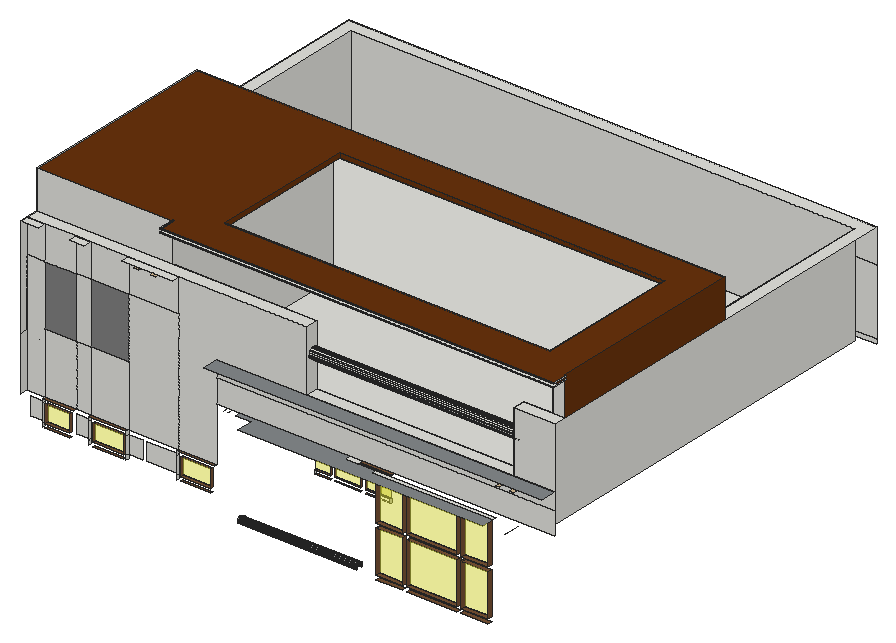
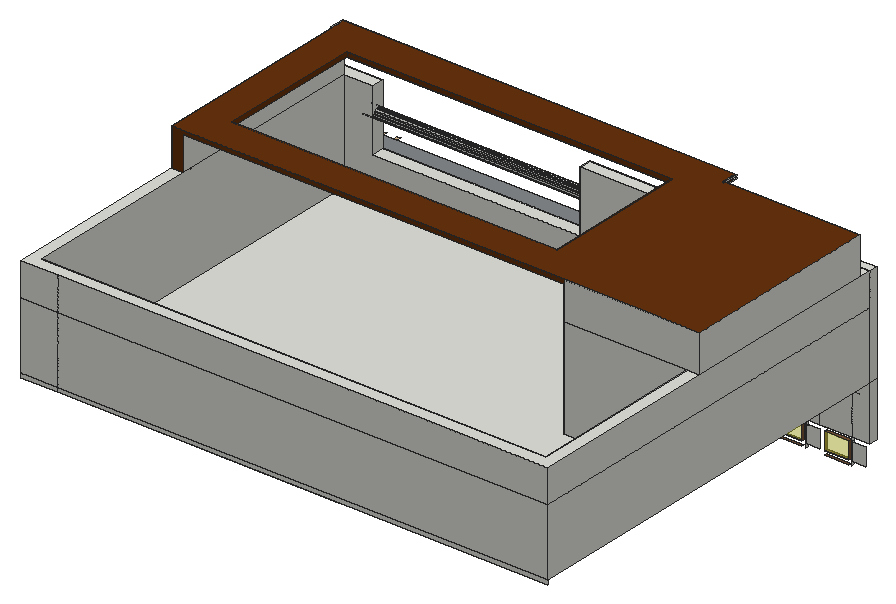
# SketchUp Ruby script. Lengths in inches.
U = 1.inch
M = Sketchup.active_model
def pt(a) = Geom::Point3d.new(a.map { |v| v * U })
def face(e, loops, mat)
  f = e.add_face(loops[0].map { |a| pt(a) })
  loops[1..].each { |l| e.add_face(l.map { |a| pt(a) }).erase! }
  f.material = f.back_material = mat if mat
  f
end
# faces: each face lists its corners as indices into pts; further lists are holes
def faces(e, pts, list, mat = nil) = list.each { |f| face(e, (f[0].is_a?(Array) ? f : [f]).map { |l| l.map { |i| pts[i] } }, mat) }
# xy, xz, yz: faces in a plane at the given z, y or x. An outline is a flat list of corners, or four numbers for a rectangle; further outlines are holes
def ring(l) = l.size == 4 ? [[l[0], l[1]], [l[2], l[1]], [l[2], l[3]], [l[0], l[3]]] : l.each_slice(2).to_a
def flat(e, list, mat, &to3) = list.each { |f| face(e, (f[0].is_a?(Array) ? f : [f]).map { |l| ring(l).map { |u, v| to3.(u, v) } }, mat) }
def xy(e, z, list, mat = nil) = flat(e, list, mat) { |x, y| [x, y, z] }
def xz(e, y, list, mat = nil) = flat(e, list, mat) { |x, z| [x, y, z] }
def yz(e, x, list, mat = nil) = flat(e, list, mat) { |y, z| [x, y, z] }
def lines(e, pts, list) = list.each { |a, b| e.add_line(pt(pts[a]), pt(pts[b])) }
# prism: a flat outline (further loops are holes) pulled along v
def prism(e, loops, v, mat = nil)
  f = face(e, loops, mat); d = Geom::Vector3d.new(v.map { |x| x * U })
  f.pushpull(f.normal.samedirection?(d) ? d.length : -d.length)
end
def box(e, o, s, mat = nil) = prism(e, [[o, [o[0] + s[0], o[1], o[2]], [o[0] + s[0], o[1] + s[1], o[2]], [o[0], o[1] + s[1], o[2]]]], [0, 0, s[2]], mat)
def at(x, y, z, deg = 0) = Geom::Transformation.translation(pt([x, y, z])) * Geom::Transformation.rotation(ORIGIN, Z_AXIS, deg.degrees)
def axes(o, x, y, z) = Geom::Transformation.new([*x, 0, *y, 0, *z, 0, *pt(o).to_a, 1])
def part(name) = M.definitions.add(name)
# library, detail: a bought-in or finely detailed component or shape, given as its bounding box
def library(name, o, s) = part(name).tap { |d| box(d.entities, o, s) }
def detail(e, o, s) = box(e.add_group.entities, o, s)
def put(e, d, t, mat = nil) = e.add_instance(d, t).tap { |i| i.material = mat if mat }
def group(e, t, mat = nil) = e.add_group.tap { |g| g.transformation = t; g.material = mat if mat }.entities
root = M.entities
M.materials.add("[0033_NavajoWhite]").color = [214, 186, 145]
M.materials.add("[0043_SaddleBrown]").color = [104, 51, 14]
M.materials.add("[0132_LightGray]").color = [169, 169, 169]
M.materials.add("[0133_Gray]").color = [128, 128, 128]
M.materials.add("[Blacktop Old 01]").color = [132, 136, 139]
M.materials.add("[Sandstone]").color = [118, 81, 52]
M.materials.add("[Translucent Glass Blue]").color = [254, 255, 58]
M.materials["[Translucent Glass Blue]"].alpha = 0.5
M.materials.add("[Wood Veneer 01]").color = [120, 70, 37]
xy(root,175.36,[[252.13,104.5,270.95,107.5],[273.95,104.5,309.9,107.5],[312.9,104.5,332.27,107.5]],"[Sandstone]")
xy(root,178.36,[[252.13,104.5,270.95,107.5],[273.95,104.5,309.9,107.5],[312.9,104.5,332.27,107.5]],"[Sandstone]")
xy(root,186.83,[[198.65,161.625,205.9,162.625],[208.9,161.625,216.46,162.625]],"[Sandstone]")
xy(root,186.83,[[162.46,161.625,173.59,162.625],[176.59,161.625,195.65,162.625]],"[Wood Veneer 01]")
xy(root,188.6,[[14.63,105.5,32.375,107.5],[48.83,105.5,70.95,107.5],[111.24,105.5,132.89,107.5]],"[Sandstone]")
xy(root,189.41,[[162.46,161.625,173.59,162.625],[176.59,161.625,195.65,162.625],[198.65,161.625,205.9,162.625],[208.9,161.625,216.46,162.625]],"[Sandstone]")
xy(root,191.6,[[14.63,105.5,32.375,107.5],[48.83,105.5,70.95,107.5],[111.24,105.5,132.89,107.5]],"[Sandstone]")
xy(root,204,[[173.59,161.625,176.59,162.625],[195.65,161.625,198.65,162.625],[205.9,161.625,208.9,162.625]])
xy(root,204,[[162.46,159.625,162.46,162.625,173.59,162.625,173.59,161.625,176.59,161.625,176.59,162.625,195.65,162.625,195.65,161.625,198.65,161.625,198.65,162.625,205.9,162.625,205.9,161.625,208.9,161.625,208.9,162.625,216.46,162.625,216.46,159.625]],"[Wood Veneer 01]")
xy(root,204.1,[[14.63,105.5,32.375,107.5],[48.83,105.5,70.95,107.5],[111.24,105.5,132.89,107.5]],"[Sandstone]")
xy(root,207,[[159.46,159.625,219.46,162.625]],"[Sandstone]")
xy(root,207.1,[[12.9375,105.5,35.3125,107.5],[45.625,105.5,72.45,107.5],[108.79,105.5,135.89,107.5]],"[Sandstone]")
xy(root,208.5625,[[252.13,104.5,270.95,107.5],[273.95,104.5,309.9,107.5],[312.9,104.5,332.27,107.5]],"[Sandstone]")
xy(root,211.5625,[[252.13,104.5,270.95,107.5],[273.95,104.5,309.9,107.5],[312.9,104.5,332.27,107.5]],"[Sandstone]")
xy(root,240,[[252.13,104.5,270.95,107.5],[273.95,104.5,309.9,107.5],[312.9,104.5,332.27,107.5]],"[Sandstone]")
xy(root,243,[[249.13,104.5,335.27,107.5],[227.6875,107.5,236.6875,162.625],[9,116.5,143.5625,162.625],[143.5625,116.5,149.5625,162.625],[9,162.625,143.5625,385.8125],
  [143.5625,162.625,143.5625,394.8125,149.5625,394.8125,149.5625,171.625,227.6875,171.625,227.6875,394.8125,236.6875,394.8125,236.6875,162.625],[149.5625,171.625,227.6875,385.8125],[9,385.8125,143.5625,394.8125],[149.5625,385.8125,227.6875,394.8125],[236.6875,385.8125,245.6875,394.8125],
  [245.6875,385.8125,351,394.8125]])
xy(root,243,[[160.6875,95.5,160.6875,107.5,149.5625,107.5,149.5625,162.625,227.6875,162.625,227.6875,107.5,249.13,107.5,249.13,104.5,335.27,104.5,335.27,95.5]],"[Blacktop Old 01]")
xy(root,246,[[97.0625,116.5,369,116.5,369,385.8125,9,385.8125,9,259.41,97.0625,259.41]])
xy(root,274.3125,[[200.18,107.5,347.95,116.5]])
xy(root,274.3125,[[347.36,92.5,350.01,95.5],[357.24,92.5,359.89,95.5]],"[0033_NavajoWhite]")
xy(root,274.3125,[[135.89,95.5,377.5,107.5]],"[Blacktop Old 01]")
xy(root,318,[[0,101.5,12.9375,107.5],[35.3125,101.5,45.625,107.5],[72.45,101.5,108.79,107.5],[0,107.5,200.18,116.5],[347.95,107.5,377.5,116.5],
  [369,116.5,377.5,259.41],[0,259.41,9,259.41,9,385.8125,369,385.8125,369,259.41,377.5,259.41,377.5,394.8125,0,394.8125]])
xy(root,318,[[82.86,99.5,86.5,101.5],[94.93,99.5,98.5625,101.5]],"[0033_NavajoWhite]")
xy(root,341.25,[[[102.89,111.64,363.17,253.59],[105.89,114.64,360.17,250.59]]])
xy(root,342.25,[[[102.89,111.64,363.17,253.59],[105.89,114.64,360.17,250.59]]])
xy(root,342.25,[[[96,105.8125,96,116.875,97.0625,116.875,97.0625,259.41,369,259.41,369,116.5,378,116.5,378,105.8125],[102.89,111.64,363.17,253.59]],[[105.89,114.64,360.17,250.59],[121.0625,132.8125,353.5,235.41]]],"[0043_SaddleBrown]")
xy(root,342.89,[[96,105.8125,378,105.8125,378,116.5,377.5,116.5,377.5,108.8125,97.0625,108.8125,97.0625,116.875,96,116.875]])
xy(root,344.5625,[[96.0625,105.8125,96.0625,117.375,97.0625,117.375,97.0625,108.8125,377.5,108.8125,377.5,116.5,377.9375,116.5,377.9375,105.8125]])
xy(root,345.2,[[96.0625,116.5,97.0625,117.375]])
xy(root,345.25,[[[96.0625,105.8125,377.9375,105.8125,377.9375,116.5,377.5,116.5,377.5,259.41,0,259.41,0,116.5,96.0625,116.5],[121.0625,132.8125,353.5,235.41]]],"[0043_SaddleBrown]")
xz(root,105.8125,[[96,342.25,378,342.89],[96.0625,344.5625,377.9375,345.25]])
xz(root,107.5,[[3,191.6,12.9375,204.1],[35.375,191.6,45.625,204.1],[72.45,191.6,82.75,204.1],[85.75,191.6,108.79,204.1],[0,207.1,12.9375,294],
  [12.9375,207.1,35.3125,250.55],[35.3125,207.1,45.625,250.55],[45.625,207.1,72.45,250.55],[72.45,207.1,108.79,294],[108.79,207.1,135.89,207.1,135.89,274.3125,200.18,274.3125,200.18,318,108.79,318],
  [135.89,246,377.5,262.3125],[35.3125,250.55,45.625,294],[135.89,262.3125,377.5,274.3125],[347.95,274.3125,377.5,318],[0,294,12.9375,318],
  [12.9375,294,35.3125,318],[35.3125,294,45.625,318],[45.625,294,72.45,318],[72.45,294,108.79,318]])
xz(root,107.5,[[12.9375,250.55,35.3125,294],[45.625,250.55,72.45,294]],"[0133_Gray]")
xz(root,107.5,[[252.13,178.36,270.95,208.5625],[273.95,178.36,309.9,208.5625],[312.9,178.36,332.27,208.5625],[14.63,191.6,32.375,204.1],[48.83,191.6,70.95,204.1],
  [111.24,191.6,132.89,204.1],[252.13,211.5625,270.95,240],[273.95,211.5625,309.9,240],[312.9,211.5625,332.27,240]],"[Translucent Glass Blue]")
xz(root,108.8125,[[97.0625,342.89,377.5,344.5625]],"[0043_SaddleBrown]")
xz(root,111.64,[[102.89,341.25,363.17,342.25]])
xz(root,114.64,[[105.89,341.25,360.17,342.25]])
xz(root,116.5,[[97.0625,246,97.0625,318,200.18,318,200.18,274.3125,347.95,274.3125,347.95,318,369,318,369,246],[0,318,97.0625,318,97.0625,345.2,96.0625,345.2,96.0625,345.25,0,345.25],[369,318,377.5,342.25],[377.5,342.25,378,342.89],[377.5,344.5625,377.9375,345.25]])
xz(root,116.875,[[96,342.25,97.0625,342.89]])
xz(root,117.375,[[96.0625,344.5625,97.0625,345.2]])
xz(root,132.8125,[[121.0625,342.25,353.5,345.25]],"[0043_SaddleBrown]")
xz(root,162.625,[[162.46,189.41,173.59,204],[176.59,189.41,195.65,204],[198.65,189.41,205.9,204],[208.9,189.41,216.46,204]],"[Translucent Glass Blue]")
xz(root,235.41,[[121.0625,342.25,353.5,345.25]],"[0043_SaddleBrown]")
xz(root,250.59,[[105.89,341.25,360.17,342.25]])
xz(root,253.59,[[102.89,341.25,363.17,342.25]])
xz(root,259.41,[[9,246,97.0625,318],[0,318,97.0625,345.25]])
xz(root,259.41,[[369,318,369,342.25,97.0625,342.25,97.0625,345.25,377.5,345.25,377.5,318]],"[0043_SaddleBrown]")
xz(root,385.8125,[[9,246,369,318]])
xz(root,394.8125,[[0,243,351,246],[351,243,377.5,246],[0,246,351,294],[351,246,377.5,294],[0,294,351,318],
  [351,294,377.5,318]])
yz(root,0,[[101.5,207.1,107.5,246],[101.5,246,107.5,318],[107.5,246,394.8125,294],[107.5,294,394.8125,318],[116.5,318,259.41,345.25]])
yz(root,9,[[259.41,246,385.8125,318]])
yz(root,12.9375,[[105.5,188.6,107.5,191.6],[105.5,191.6,107.5,204.1],[105.5,204.1,107.5,207.1]])
yz(root,14.63,[[105.5,191.6,107.5,204.1]],"[Sandstone]")
yz(root,32.375,[[105.5,191.6,107.5,204.1]],"[Sandstone]")
yz(root,45.625,[[105.5,188.6,107.5,191.6],[105.5,191.6,107.5,204.1],[105.5,204.1,107.5,207.1]])
yz(root,48.83,[[105.5,191.6,107.5,204.1]],"[Sandstone]")
yz(root,70.95,[[105.5,191.6,107.5,204.1]],"[Sandstone]")
yz(root,72.45,[[105.5,188.6,107.5,191.6],[105.5,191.6,107.5,204.1],[105.5,204.1,107.5,207.1]])
yz(root,96,[[105.8125,342.25,116.875,342.89]])
yz(root,96.0625,[[105.8125,344.5625,105.8125,345.25,116.5,345.25,116.5,345.2,117.375,345.2,117.375,344.5625]])
yz(root,97.0625,[[116.5,246,259.41,342.25],[116.5,342.25,116.875,342.89],[108.8125,344.5625,116.5,345.2],[116.5,344.5625,117.375,345.2],[108.8125,345.2,116.5,345.25]])
yz(root,97.0625,[[108.8125,342.89,116.5,344.5625]],"[0043_SaddleBrown]")
yz(root,102.89,[[111.64,341.25,253.59,342.25]])
yz(root,105.89,[[114.64,341.25,250.59,342.25]])
yz(root,108.79,[[105.5,188.6,107.5,191.6],[105.5,191.6,107.5,204.1],[105.5,204.1,107.5,207.1]])
yz(root,111.24,[[105.5,191.6,107.5,204.1]],"[Sandstone]")
yz(root,121.0625,[[132.8125,342.25,235.41,345.25]],"[0043_SaddleBrown]")
yz(root,132.89,[[105.5,191.6,107.5,204.1]],"[Sandstone]")
yz(root,162.46,[[161.625,186.83,162.625,189.41]])
yz(root,173.59,[[161.625,189.41,162.625,204]],"[Sandstone]")
yz(root,176.59,[[161.625,189.41,162.625,204]],"[Sandstone]")
yz(root,195.65,[[161.625,189.41,162.625,204]],"[Sandstone]")
yz(root,198.65,[[161.625,189.41,162.625,204]],"[Sandstone]")
yz(root,200.18,[[[107.5,274.3125,116.5,318],[112.5,295.76,111.53,295.89,110.63,296.26,109.85,296.86,109.26,297.63,108.88,298.54,108.75,299.51,108.88,300.48,109.26,301.38,109.85,302.16,110.63,302.75,111.53,303.13,112.5,303.26,113.47,303.13,114.38,302.75,115.15,302.16,115.75,301.38,116.125,300.48,116.25,299.51,116.125,298.54,115.75,297.63,115.15,296.86,114.38,296.26,113.47,295.89]]])
yz(root,205.9,[[161.625,189.41,162.625,204]],"[Sandstone]")
yz(root,208.9,[[161.625,189.41,162.625,204]],"[Sandstone]")
yz(root,216.46,[[161.625,186.83,162.625,189.41]])
yz(root,252.13,[[104.5,178.36,107.5,208.5625],[104.5,211.5625,107.5,240]],"[Sandstone]")
yz(root,270.95,[[104.5,178.36,107.5,208.5625],[104.5,211.5625,107.5,240]],"[Sandstone]")
yz(root,273.95,[[104.5,178.36,107.5,208.5625],[104.5,211.5625,107.5,240]],"[Sandstone]")
yz(root,309.9,[[104.5,178.36,107.5,208.5625],[104.5,211.5625,107.5,240]],"[Sandstone]")
yz(root,312.9,[[104.5,178.36,107.5,208.5625],[104.5,211.5625,107.5,240]],"[Sandstone]")
yz(root,332.27,[[104.5,178.36,107.5,208.5625],[104.5,211.5625,107.5,240]],"[Sandstone]")
yz(root,347.95,[[107.5,274.3125,116.5,318]])
yz(root,353.5,[[132.8125,342.25,235.41,345.25]],"[0043_SaddleBrown]")
yz(root,356.36,[[112.5,295.76,113.47,295.89,114.38,296.26,115.15,296.86,115.75,297.63,116.125,298.54,116.25,299.51,116.125,300.48,115.75,301.38,115.15,302.16,114.38,302.75,113.47,303.13,112.5,303.26,111.53,303.13,110.63,302.75,109.85,302.16,109.26,301.38,108.88,300.48,108.75,299.51,108.88,298.54,109.26,297.63,109.85,296.86,110.63,296.26,111.53,295.89]])
yz(root,360.17,[[114.64,341.25,250.59,342.25]])
yz(root,363.17,[[111.64,341.25,253.59,342.25]])
yz(root,369,[[116.5,246,385.8125,318],[116.5,318,259.41,342.25]])
yz(root,377.5,[[116.5,318,259.41,318,259.41,345.25,116.5,345.25,116.5,344.5625,108.8125,344.5625,108.8125,342.89,116.5,342.89]],"[0043_SaddleBrown]")
yz(root,377.9375,[[105.8125,344.5625,116.5,345.25]])
yz(root,378,[[105.8125,342.25,116.5,342.89]])
p = [[149.5625,109.11,174.27],[149.5625,109.35,173.68],[234.5625,109.35,173.68],[234.5625,109.11,174.27],[149.5625,113.57,173.68],[149.5625,113.8125,174.27],
  [234.5625,113.8125,174.27],[234.5625,113.57,173.68],[149.5625,109.02,174.9],[234.5625,109.02,174.9],[149.5625,113.9,174.9],[234.5625,113.9,174.9],
  [149.5625,109.11,175.53],[234.5625,109.11,175.53],[149.5625,113.8125,175.53],[234.5625,113.8125,175.53],[149.5625,109.35,176.12],[234.5625,109.35,176.12],
  [149.5625,113.57,176.12],[234.5625,113.57,176.12],[149.5625,109.74,176.62],[234.5625,109.74,176.62],[149.5625,113.18,176.62],[234.5625,113.18,176.62],
  [149.5625,110.24,177.01],[234.5625,110.24,177.01],[149.5625,112.68,177.01],[234.5625,112.68,177.01],[149.5625,110.83,177.25],[234.5625,110.83,177.25],
  [149.5625,112.09,177.25],[234.5625,112.09,177.25],[149.5625,111.46,177.34],[234.5625,111.46,177.34],[200.18,111.53,295.89],[200.18,112.5,295.76],
  [356.36,112.5,295.76],[356.36,111.53,295.89],[200.18,113.47,295.89],[356.36,113.47,295.89],[200.18,110.63,296.26],[356.36,110.63,296.26],
  [200.18,114.38,296.26],[356.36,114.38,296.26],[200.18,109.85,296.86],[356.36,109.85,296.86],[200.18,115.15,296.86],[356.36,115.15,296.86],
  [200.18,109.26,297.63],[356.36,109.26,297.63],[200.18,115.75,297.63],[356.36,115.75,297.63],[200.18,108.88,298.54],[356.36,108.88,298.54],
  [200.18,116.125,298.54],[356.36,116.125,298.54],[200.18,108.75,299.51],[356.36,108.75,299.51],[200.18,116.25,299.51],[356.36,116.25,299.51],
  [200.18,108.88,300.48],[356.36,108.88,300.48],[200.18,116.125,300.48],[356.36,116.125,300.48],[200.18,109.26,301.38],[356.36,109.26,301.38],
  [200.18,115.75,301.38],[356.36,115.75,301.38],[200.18,109.85,302.16],[356.36,109.85,302.16],[200.18,115.15,302.16],[356.36,115.15,302.16],
  [200.18,110.63,302.75],[356.36,110.63,302.75],[200.18,114.38,302.75],[356.36,114.38,302.75],[200.18,111.53,303.13],[356.36,111.53,303.13],
  [200.18,113.47,303.13],[356.36,113.47,303.13],[200.18,112.5,303.26],[356.36,112.5,303.26],[9,116.5,243],[0,116.5,243],
  [9,162.625,243],[0,162.625,243],[9,107.5,243],[140.5625,116.5,243],[140.5625,107.5,243],[143.5625,116.5,243],
  [143.5625,107.5,243],[236.6875,116.5,243],[360,116.5,243],[351,107.5,243],[351,95.5,243],[97.0625,108.8125,342.25],
  [97.0625,108.8125,342.89],[97.0625,108.8125,345.2],[96.0625,108.8125,345.2],[97.0625,116.5,345.25],[96.0625,116.5,345.25]]
faces(root,p,[[0,1,2,3],[4,5,6,7],[8,0,3,9],[5,10,11,6],[12,8,9,13],[10,14,15,11],[16,12,13,17],[14,18,19,15],
  [20,16,17,21],[18,22,23,19],[24,20,21,25],[22,26,27,23],[28,24,25,29],[26,30,31,27],[32,28,29,33],[30,32,33,31]],"[0132_LightGray]")
faces(root,p,[[34,35,36,37],[35,38,39,36],[40,34,37,41],[38,42,43,39],[44,40,41,45],[42,46,47,43],[48,44,45,49],[46,50,51,47],
  [52,48,49,53],[50,54,55,51],[56,52,53,57],[54,58,59,55],[60,56,57,61],[58,62,63,59],[64,60,61,65],[62,66,67,63],
  [68,64,65,69],[66,70,71,67],[72,68,69,73],[70,74,75,71],[76,72,73,77],[74,78,79,75],[80,76,77,81],[78,80,81,79]])
lines(root,p,[[82,83],[84,85],[82,86],[87,88],[89,90],[91,92],[93,94],[95,96],[97,98],[99,100]])
